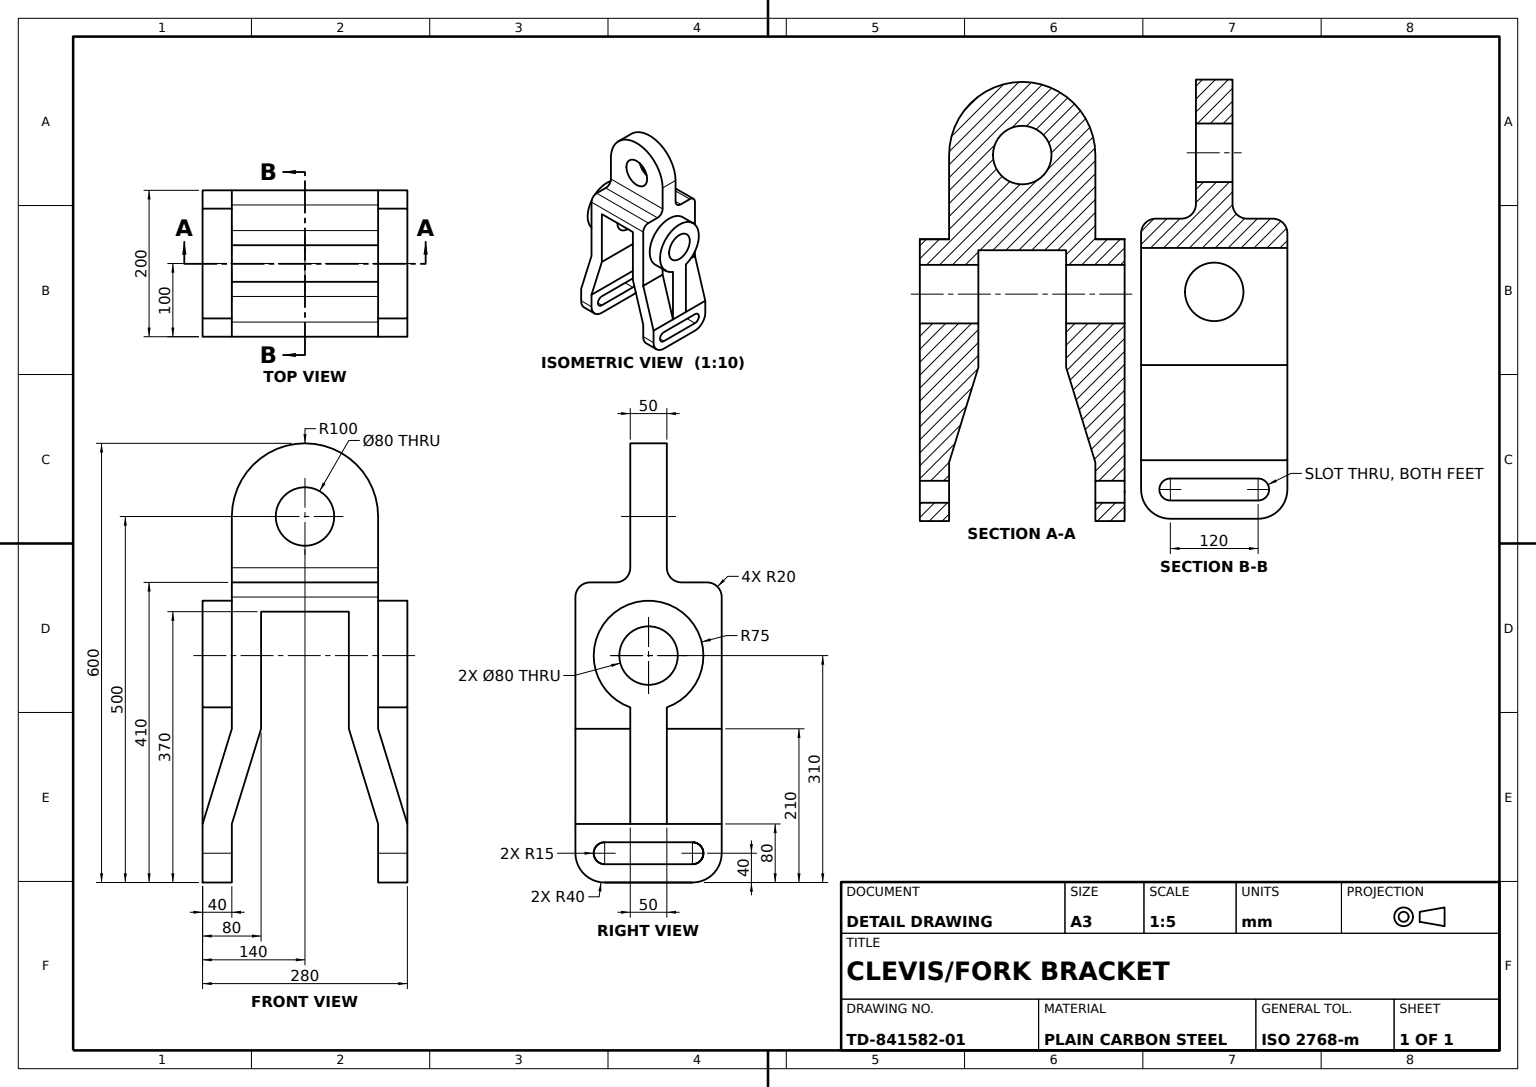
solid
v1 (139.993222,-330,-200)
v2 (100,-200,-200)
e1 v1 v2 LINE
v3 (100,-200,-125)
e2 v2 v3 LINE
v4 (139.993222,-330,-125)
e3 v4 v3 LINE
e4 v1 v4 LINE
face PLANE(AX(P(100,-200,-200),D(0.955793015,0.294040325,0),D(-0.294040325,0.955793015,0))) [e1 e2 -e3 -e4]
v5 (60,-100,-60)
v6 (140,-100,-60)
e5 v5 v6 LINE
v7 (140,-100,-140)
e6 v6 v7 CIRCLE(AX(P(140,-100,-100),D(1,0,0),D(0,0,-1)),40)
v8 (60,-100,-140)
e7 v8 v7 LINE
e8 v8 v5 CIRCLE(AX(P(60,-100,-100),D(-1,0,0),D(0,0,1)),40)
face CYL(AX(P(100,-100,-100),D(1,0,0),D(0,0,-1)),40) rev [e5 e6 -e7 e8]
v9 (-100,-100,-175)
v10 (-100,-100,-25)
e9 v9 v10 CIRCLE(AX(P(-100,-100,-100),D(1,0,0),D(0,0,-1)),75)
v11 (-140,-100,-175)
e10 v9 v11 LINE
v12 (-140,-100,-25)
e11 v11 v12 CIRCLE(AX(P(-140,-100,-100),D(1,0,0),D(0,0,-1)),75)
e12 v10 v12 LINE
face CYL(AX(P(-100,-100,-100),D(-1,0,0),D(0,0,1)),75) [-e9 e10 e11 -e12]
v13 (-100,0,-55)
v14 (-100,20,-75)
e13 v13 v14 CIRCLE(AX(P(-100,20,-55),D(1,0,0),D(0,0,1)),20)
v15 (100,0,-55)
e14 v15 v13 LINE
v16 (100,20,-75)
e15 v16 v15 CIRCLE(AX(P(100,20,-55),D(-1,0,0),D(0,0,-1)),20)
e16 v14 v16 LINE
face CYL(AX(P(0,20,-55),D(-1,0,0),D(0,0,1)),20) rev [-e13 -e14 -e15 -e16]
v17 (60,-40,-200)
v18 (60,-200,-200)
e17 v17 v18 LINE
v19 (60,-200,0)
e18 v18 v19 LINE
v20 (60,-40,0)
e19 v20 v19 LINE
e20 v17 v20 LINE
e21 v5 v8 CIRCLE(AX(P(60,-100,-100),D(-1,0,0),D(0,0,1)),40)
face PLANE(AX(P(60,-200,-200),D(-1,0,0),D(0,0,1))) [e17 e18 -e19 -e20] [-e8 -e21]
v21 (139.993222,-370,-200)
v22 (99.993222,-370,-200)
e22 v21 v22 LINE
v23 (139.993222,-410,-160)
e23 v23 v21 CIRCLE(AX(P(139.993222,-370,-160),D(1,0,0),D(0,0,-1)),40)
v24 (99.993222,-410,-160)
e24 v24 v23 LINE
e25 v22 v24 CIRCLE(AX(P(99.993222,-370,-160),D(-1,0,0),D(0,0,1)),40)
face CYL(AX(P(0,-370,-160),D(-1,0,0),D(0,0,1)),40) [-e22 -e23 -e24 -e25]
v25 (-100,0,-20)
e26 v13 v25 LINE
v26 (100,0,-20)
e27 v25 v26 LINE
e28 v15 v26 LINE
face PLANE(AX(P(0,0,-200),D(0,1,0),D(0,0,1))) [e26 e27 -e28 e14]
v27 (-99.993222,-370,-200)
v28 (-139.993222,-370,-200)
e29 v27 v28 LINE
v29 (-99.993222,-410,-160)
e30 v29 v27 CIRCLE(AX(P(-99.993222,-370,-160),D(1,0,0),D(0,0,-1)),40)
v30 (-139.993222,-410,-160)
e31 v30 v29 LINE
e32 v28 v30 CIRCLE(AX(P(-139.993222,-370,-160),D(-1,0,0),D(0,0,1)),40)
face CYL(AX(P(0,-370,-160),D(-1,0,0),D(0,0,1)),40) [-e29 -e30 -e31 -e32]
v31 (-99.993222,-410,-40)
e33 v29 v31 LINE
v32 (-139.993222,-410,-40)
e34 v31 v32 LINE
e35 v30 v32 LINE
face PLANE(AX(P(-139.993222,-410,-200),D(0,-1,0),D(0,0,-1))) [e31 e33 e34 -e35]
v33 (-60,-200,-200)
v34 (-60,-200,0)
e36 v33 v34 LINE
v35 (-99.993222,-330,0)
e37 v35 v34 LINE
v36 (-99.993222,-330,-200)
e38 v36 v35 LINE
e39 v36 v33 LINE
face PLANE(AX(P(-99.993222,-330,-200),D(0.955793015,-0.294040325,0),D(0.294040325,0.955793015,0))) [e36 -e37 -e38 e39]
v37 (100,-200,-75)
v38 (139.993222,-330,-75)
e40 v37 v38 LINE
v39 (100,-200,0)
e41 v37 v39 LINE
v40 (139.993222,-330,0)
e42 v40 v39 LINE
e43 v38 v40 LINE
face PLANE(AX(P(100,-200,-200),D(0.955793015,0.294040325,0),D(-0.294040325,0.955793015,0))) [-e40 e41 -e42 -e43]
v41 (140,-170.710678,-125)
v42 (140,-100,-175)
e44 v41 v42 CIRCLE(AX(P(140,-100,-100),D(1,0,0),D(0,0,-1)),75)
v43 (100,-170.710678,-125)
e45 v43 v41 LINE
v44 (100,-100,-175)
e46 v43 v44 CIRCLE(AX(P(100,-100,-100),D(1,0,0),D(0,0,-1)),75)
e47 v44 v42 LINE
face CYL(AX(P(100,-100,-100),D(1,0,0),D(0,0,-1)),75) [-e44 -e45 e46 e47]
v45 (100,-170.710678,-75)
v46 (140,-170.710678,-75)
e48 v45 v46 LINE
e49 v45 v37 LINE
v47 (140,-330,-75)
e50 v38 v47 LINE
e51 v46 v47 LINE
face PLANE(AX(P(100,-170.710678,-75),D(0,0,1),D(0,-1,0))) [-e48 e49 e40 e50 -e51]
v48 (99.993222,-385,-160)
v49 (139.993222,-385,-160)
e52 v48 v49 LINE
v50 (99.993222,-385,-40)
e53 v48 v50 LINE
v51 (139.993222,-385,-40)
e54 v50 v51 LINE
e55 v51 v49 LINE
face PLANE(AX(P(-140,-385,-40),D(0,-1,0),D(0,0,-1))) rev [-e52 e53 e54 e55]
v52 (40,90,-75)
v53 (-40,90,-75)
e56 v52 v53 CIRCLE(AX(P(0,90,-75),D(0,0,1),D(1,0,0)),40)
v54 (-40,90,-125)
e57 v53 v54 LINE
v55 (40,90,-125)
e58 v55 v54 CIRCLE(AX(P(0,90,-125),D(0,0,1),D(1,0,0)),40)
e59 v52 v55 LINE
face CYL(AX(P(0,90,-75),D(0,0,-1),D(-1,0,0)),40) rev [e56 e57 -e58 -e59]
v56 (-99.993222,-355,-40)
v57 (-99.993222,-385,-40)
e60 v56 v57 CIRCLE(AX(P(-99.993222,-370,-40),D(1,0,0),D(0,0,-1)),15)
v58 (-99.993222,-355,-160)
e61 v58 v56 LINE
v59 (-99.993222,-370,-175)
e62 v59 v58 CIRCLE(AX(P(-99.993222,-370,-160),D(1,0,0),D(0,0,-1)),15)
v60 (-99.993222,-385,-160)
e63 v60 v59 CIRCLE(AX(P(-99.993222,-370,-160),D(1,0,0),D(0,0,-1)),15)
e64 v57 v60 LINE
v61 (-99.993222,-370,0)
e65 v61 v31 CIRCLE(AX(P(-99.993222,-370,-40),D(1,0,0),D(0,0,-1)),40)
e66 v27 v36 LINE
e67 v61 v35 LINE
face PLANE(AX(P(-99.993222,-410,-200),D(1,0,0),D(0,0,-1))) [-e60 -e61 -e62 -e63 -e64] [e65 -e33 e30 e66 e38 -e67]
v62 (139.993222,-410,-40)
e68 v23 v62 LINE
v63 (99.993222,-410,-40)
e69 v62 v63 LINE
e70 v24 v63 LINE
face PLANE(AX(P(139.993222,-410,-200),D(0,-1,0),D(0,0,-1))) [e68 e69 -e70 e24]
v64 (-139.993222,-385,-160)
v65 (-139.993222,-385,-40)
e71 v64 v65 LINE
v66 (-139.993222,-370,-175)
e72 v66 v64 CIRCLE(AX(P(-139.993222,-370,-160),D(-1,0,0),D(0,0,1)),15)
v67 (-139.993222,-355,-160)
e73 v67 v66 CIRCLE(AX(P(-139.993222,-370,-160),D(-1,0,0),D(0,0,1)),15)
v68 (-139.993222,-355,-40)
e74 v68 v67 LINE
e75 v65 v68 CIRCLE(AX(P(-139.993222,-370,-40),D(-1,0,0),D(0,0,1)),15)
v69 (-139.993222,-370,0)
e76 v32 v69 CIRCLE(AX(P(-139.993222,-370,-40),D(-1,0,0),D(0,0,1)),40)
v70 (-139.993222,-330,0)
e77 v70 v69 LINE
v71 (-139.993222,-330,-75)
e78 v71 v70 LINE
v72 (-139.993222,-330,-125)
e79 v72 v71 LINE
v73 (-139.993222,-330,-200)
e80 v73 v72 LINE
e81 v73 v28 LINE
face PLANE(AX(P(-139.993222,-330,-200),D(-1,0,0),D(0,0,1))) [-e71 -e72 -e73 -e74 -e75] [e76 -e77 -e78 -e79 -e80 e81 e32 e35]
v74 (99.993222,-330,-200)
e82 v18 v74 LINE
v75 (99.993222,-330,0)
e83 v74 v75 LINE
e84 v19 v75 LINE
face PLANE(AX(P(99.993222,-330,-200),D(-0.955793015,-0.294040325,0),D(0.294040325,-0.955793015,0))) [-e18 e82 e83 -e84]
v76 (-100,-170.710678,-125)
e85 v76 v9 CIRCLE(AX(P(-100,-100,-100),D(1,0,0),D(0,0,-1)),75)
v77 (-140,-170.710678,-125)
e86 v76 v77 LINE
e87 v77 v11 CIRCLE(AX(P(-140,-100,-100),D(1,0,0),D(0,0,-1)),75)
face CYL(AX(P(-100,-100,-100),D(-1,0,0),D(0,0,1)),75) [-e85 e86 e87 -e10]
v78 (-140,-330,-125)
e88 v72 v78 LINE
e89 v78 v77 LINE
v79 (-100,-200,-125)
e90 v79 v76 LINE
e91 v72 v79 LINE
face PLANE(AX(P(-100,-170.710678,-125),D(0,0,1),D(0,-1,0))) rev [e88 e89 -e86 -e90 -e91]
e92 v66 v59 LINE
e93 v67 v58 LINE
face CYL(AX(P(-140,-370,-160),D(1,0,0),D(0,0,-1)),15) rev [e73 e92 e62 -e93]
v80 (-100,90,-75)
v81 (-100,90,-125)
e94 v80 v81 LINE
v82 (-100,20,-125)
e95 v81 v82 LINE
v83 (-100,0,-145)
e96 v82 v83 CIRCLE(AX(P(-100,20,-145),D(1,0,0),D(0,0,1)),20)
v84 (-100,0,-180)
e97 v84 v83 LINE
v85 (-100,-20,-200)
e98 v84 v85 CIRCLE(AX(P(-100,-20,-180),D(-1,0,0),D(0,0,1)),20)
v86 (-100,-200,-200)
e99 v85 v86 LINE
e100 v86 v79 LINE
v87 (-100,-170.710678,-75)
e101 v10 v87 CIRCLE(AX(P(-100,-100,-100),D(1,0,0),D(0,0,-1)),75)
v88 (-100,-200,-75)
e102 v87 v88 LINE
v89 (-100,-200,0)
e103 v88 v89 LINE
v90 (-100,-20,0)
e104 v90 v89 LINE
e105 v90 v25 CIRCLE(AX(P(-100,-20,-20),D(-1,0,0),D(0,0,1)),20)
e106 v80 v14 LINE
face PLANE(AX(P(-100,0,-200),D(-1,0,0),D(0,0,1))) [e94 e95 e96 -e97 e98 e99 e100 e90 e85 e9 e101 e102 e103 -e104 e105 -e26 e13 -e106]
v91 (-60,-40,0)
e107 v34 v91 LINE
e108 v91 v20 LINE
v92 (99.993222,-370,0)
e109 v75 v92 LINE
v93 (139.993222,-370,0)
e110 v92 v93 LINE
e111 v93 v40 LINE
v94 (100,-20,0)
e112 v39 v94 LINE
e113 v94 v90 LINE
e114 v89 v70 LINE
e115 v69 v61 LINE
face PLANE(AX(P(0,0,0),D(0,0,-1),D(-1,0,0))) rev [e67 e37 e107 e108 e19 e84 e109 e110 e111 e42 e112 e113 e104 e114 e77 e115]
v95 (100,90,-75)
e116 v95 v80 CIRCLE(AX(P(0,90,-75),D(0,0,1),D(1,0,0)),100)
v96 (100,90,-125)
e117 v95 v96 LINE
e118 v96 v81 CIRCLE(AX(P(0,90,-125),D(0,0,1),D(1,0,0)),100)
face CYL(AX(P(0,90,-75),D(0,0,-1),D(-1,0,0)),100) [-e94 -e116 e117 e118]
e119 v4 v38 LINE
v97 (140,-330,-125)
e120 v4 v97 LINE
e121 v47 v97 LINE
face PLANE(AX(P(100,-330,-75),D(0,-1,0),D(0,0,-1))) [-e50 -e119 e120 -e121]
v98 (139.993222,-370,-175)
v99 (139.993222,-355,-160)
e122 v98 v99 CIRCLE(AX(P(139.993222,-370,-160),D(1,0,0),D(0,0,-1)),15)
e123 v49 v98 CIRCLE(AX(P(139.993222,-370,-160),D(1,0,0),D(0,0,-1)),15)
v100 (139.993222,-355,-40)
e124 v100 v51 CIRCLE(AX(P(139.993222,-370,-40),D(1,0,0),D(0,0,-1)),15)
e125 v99 v100 LINE
e126 v93 v62 CIRCLE(AX(P(139.993222,-370,-40),D(1,0,0),D(0,0,-1)),40)
e127 v21 v1 LINE
face PLANE(AX(P(139.993222,-330,-200),D(1,0,0),D(0,0,-1))) [-e122 -e123 -e55 -e124 -e125] [-e111 e126 -e68 e23 e127 e4 e119 e43]
e128 v54 v55 CIRCLE(AX(P(0,90,-125),D(0,0,1),D(1,0,0)),40)
e129 v53 v52 CIRCLE(AX(P(0,90,-75),D(0,0,1),D(1,0,0)),40)
face CYL(AX(P(0,90,-75),D(0,0,-1),D(-1,0,0)),40) rev [-e128 -e57 e129 e59]
e130 v7 v6 CIRCLE(AX(P(140,-100,-100),D(1,0,0),D(0,0,-1)),40)
face CYL(AX(P(100,-100,-100),D(1,0,0),D(0,0,-1)),40) rev [e130 -e5 e21 e7]
e131 v68 v56 LINE
face PLANE(AX(P(-140,-355,-40),D(0,1,0),D(0,0,1))) rev [e61 -e131 e74 e93]
v101 (-60,-100,-140)
v102 (-60,-100,-60)
e132 v101 v102 CIRCLE(AX(P(-60,-100,-100),D(1,0,0),D(0,1,0)),40)
v103 (-140,-100,-60)
e133 v102 v103 LINE
v104 (-140,-100,-140)
e134 v104 v103 CIRCLE(AX(P(-140,-100,-100),D(1,0,0),D(0,0,-1)),40)
e135 v101 v104 LINE
face CYL(AX(P(-100,-100,-100),D(-1,0,0),D(0,0,1)),40) rev [e132 e133 -e134 -e135]
v105 (140,-100,-25)
e136 v105 v46 CIRCLE(AX(P(140,-100,-100),D(1,0,0),D(0,0,-1)),75)
v106 (100,-100,-25)
e137 v106 v105 LINE
e138 v106 v45 CIRCLE(AX(P(100,-100,-100),D(1,0,0),D(0,0,-1)),75)
face CYL(AX(P(100,-100,-100),D(1,0,0),D(0,0,-1)),75) [e48 -e136 -e137 e138]
v107 (-60,-40,-200)
e139 v107 v91 LINE
e140 v33 v107 LINE
e141 v102 v101 CIRCLE(AX(P(-60,-100,-100),D(1,0,0),D(0,1,0)),40)
face PLANE(AX(P(-60,-200,-200),D(1,0,0),D(0,1,0))) [e139 -e107 -e36 e140] [-e132 -e141]
v108 (99.993222,-355,-160)
e142 v108 v99 LINE
v109 (99.993222,-370,-175)
e143 v108 v109 CIRCLE(AX(P(99.993222,-370,-160),D(-1,0,0),D(0,0,1)),15)
e144 v109 v98 LINE
face CYL(AX(P(-140,-370,-160),D(1,0,0),D(0,0,-1)),15) rev [e122 -e142 e143 e144]
e145 v103 v104 CIRCLE(AX(P(-140,-100,-100),D(1,0,0),D(0,0,-1)),40)
face CYL(AX(P(-100,-100,-100),D(-1,0,0),D(0,0,1)),40) rev [e141 e135 -e145 -e133]
v110 (100,0,-145)
e146 v83 v110 LINE
v111 (100,0,-180)
e147 v111 v110 LINE
e148 v111 v84 LINE
face PLANE(AX(P(0,0,-200),D(0,1,0),D(0,0,1))) [e97 e146 -e147 e148]
v112 (-140,-170.710678,-75)
e149 v12 v112 CIRCLE(AX(P(-140,-100,-100),D(1,0,0),D(0,0,-1)),75)
e150 v87 v112 LINE
face CYL(AX(P(-100,-100,-100),D(-1,0,0),D(0,0,1)),75) [e149 -e150 -e101 e12]
e151 v97 v41 LINE
e152 v42 v105 CIRCLE(AX(P(140,-100,-100),D(1,0,0),D(0,0,-1)),75)
face PLANE(AX(P(140,-100,-100),D(1,0,0),D(0,0,-1))) [e151 e44 e152 e136 e51 e121] [-e130 -e6]
v113 (-140,-330,-75)
e153 v71 v113 LINE
e154 v113 v78 LINE
face PLANE(AX(P(-100,-330,-125),D(0,1,0),D(0,0,1))) rev [-e88 e79 e153 e154]
e155 v26 v94 CIRCLE(AX(P(100,-20,-20),D(1,0,0),D(0,0,-1)),20)
face CYL(AX(P(0,-20,-20),D(1,0,0),D(0,0,-1)),20) [-e155 -e27 -e105 -e113]
v114 (99.993222,-355,-40)
e156 v114 v100 LINE
e157 v114 v108 LINE
face PLANE(AX(P(-140,-355,-40),D(0,1,0),D(0,0,1))) rev [e142 e125 -e156 e157]
e158 v64 v60 LINE
e159 v65 v57 LINE
face PLANE(AX(P(-140,-385,-40),D(0,-1,0),D(0,0,-1))) rev [e64 -e158 e71 e159]
v115 (100,-20,-200)
e160 v115 v111 CIRCLE(AX(P(100,-20,-180),D(1,0,0),D(0,0,-1)),20)
e161 v85 v115 LINE
face CYL(AX(P(0,-20,-180),D(-1,0,0),D(0,0,1)),20) [-e98 -e148 -e160 -e161]
e162 v44 v106 CIRCLE(AX(P(100,-100,-100),D(1,0,0),D(0,0,-1)),75)
face CYL(AX(P(100,-100,-100),D(1,0,0),D(0,0,-1)),75) [e162 e137 -e152 -e47]
e163 v16 v95 LINE
face PLANE(AX(P(0,90,-75),D(0,0,1),D(1,0,0))) [e163 e116 e106 e16] [-e129 -e56]
e164 v88 v71 LINE
face PLANE(AX(P(-139.993222,-330,-200),D(-0.955793015,0.294040325,0),D(-0.294040325,-0.955793015,0))) [e78 -e114 -e103 e164]
face CYL(AX(P(-140,-370,-40),D(1,0,0),D(0,0,-1)),15) rev [e131 e60 -e159 e75]
e165 v109 v48 CIRCLE(AX(P(99.993222,-370,-160),D(-1,0,0),D(0,0,1)),15)
face CYL(AX(P(-140,-370,-160),D(1,0,0),D(0,0,-1)),15) rev [e165 e52 e123 -e144]
e166 v86 v73 LINE
e167 v2 v115 LINE
e168 v74 v22 LINE
e169 v107 v17 LINE
face PLANE(AX(P(0,0,-200),D(0,0,-1),D(-1,0,0))) [-e66 e29 -e81 -e166 -e99 e161 -e167 -e1 -e127 e22 -e168 -e82 -e17 -e169 -e140 -e39]
face CYL(AX(P(0,-370,-40),D(-1,0,0),D(0,0,1)),40) [-e34 -e65 -e115 -e76]
v116 (100,20,-125)
e170 v116 v96 LINE
e171 v116 v82 LINE
face PLANE(AX(P(0,90,-125),D(0,0,1),D(1,0,0))) rev [-e170 e171 -e95 -e118] [e58 e128]
e172 v63 v92 CIRCLE(AX(P(99.993222,-370,-40),D(-1,0,0),D(0,0,1)),40)
face CYL(AX(P(0,-370,-40),D(-1,0,0),D(0,0,1)),40) [-e110 -e172 -e69 -e126]
e173 v110 v116 CIRCLE(AX(P(100,20,-145),D(-1,0,0),D(0,0,-1)),20)
face CYL(AX(P(0,20,-145),D(1,0,0),D(0,0,-1)),20) rev [-e146 -e96 -e171 -e173]
e174 v50 v114 CIRCLE(AX(P(99.993222,-370,-40),D(-1,0,0),D(0,0,1)),15)
face CYL(AX(P(-140,-370,-40),D(1,0,0),D(0,0,-1)),15) rev [e124 -e54 e174 e156]
face PLANE(AX(P(60,-40,-200),D(0,-1,0),D(0,0,-1))) [e169 e20 -e108 -e139]
e175 v112 v113 LINE
face PLANE(AX(P(-100,-170.710678,-75),D(0,0,-1),D(0,1,0))) rev [-e102 e150 e175 -e153 -e164]
face PLANE(AX(P(-140,-100,-100),D(1,0,0),D(0,0,-1))) rev [e134 e145] [-e175 -e149 -e11 -e87 -e89 -e154]
face CYL(AX(P(-140,-370,-160),D(1,0,0),D(0,0,-1)),15) rev [e63 -e92 e72 e158]
face PLANE(AX(P(-139.993222,-330,-200),D(-0.955793015,0.294040325,0),D(-0.294040325,-0.955793015,0))) [e166 e80 e91 -e100]
face PLANE(AX(P(99.993222,-410,-200),D(-1,0,0),D(0,0,1))) [e168 e25 e70 e172 -e109 -e83] [-e143 -e157 -e174 -e53 -e165]
e176 v3 v43 LINE
face PLANE(AX(P(100,0,-200),D(1,0,0),D(0,0,-1))) [-e41 -e49 -e138 -e162 -e46 -e176 -e2 e167 e160 e147 e173 e170 -e117 -e163 e15 e28 e155 -e112]
face PLANE(AX(P(100,-170.710678,-125),D(0,0,-1),D(0,1,0))) [-e120 e3 e176 e45 -e151]
